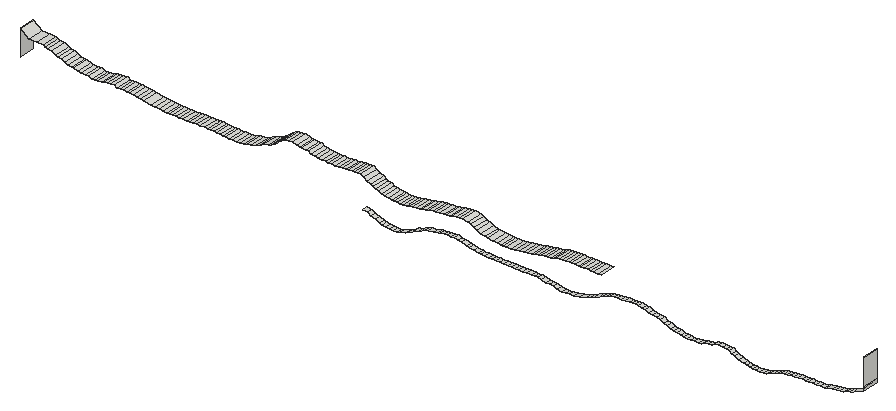
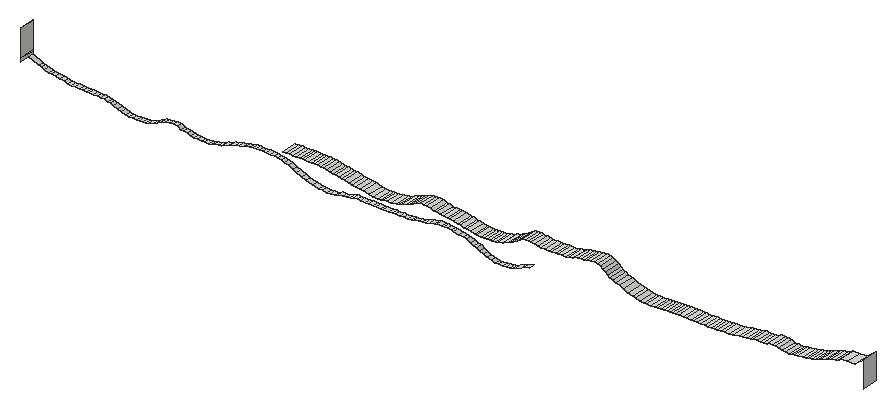
# SketchUp Ruby script. Lengths in inches.
U = 1.inch
M = Sketchup.active_model
def pt(a) = Geom::Point3d.new(a.map { |v| v * U })
def face(e, loops, mat)
  f = e.add_face(loops[0].map { |a| pt(a) })
  loops[1..].each { |l| e.add_face(l.map { |a| pt(a) }).erase! }
  f.material = f.back_material = mat if mat
  f
end
# faces: each face lists its corners as indices into pts; further lists are holes
def faces(e, pts, list, mat = nil) = list.each { |f| face(e, (f[0].is_a?(Array) ? f : [f]).map { |l| l.map { |i| pts[i] } }, mat) }
# xy, xz, yz: faces in a plane at the given z, y or x. An outline is a flat list of corners, or four numbers for a rectangle; further outlines are holes
def ring(l) = l.size == 4 ? [[l[0], l[1]], [l[2], l[1]], [l[2], l[3]], [l[0], l[3]]] : l.each_slice(2).to_a
def flat(e, list, mat, &to3) = list.each { |f| face(e, (f[0].is_a?(Array) ? f : [f]).map { |l| ring(l).map { |u, v| to3.(u, v) } }, mat) }
def xy(e, z, list, mat = nil) = flat(e, list, mat) { |x, y| [x, y, z] }
def xz(e, y, list, mat = nil) = flat(e, list, mat) { |x, z| [x, y, z] }
def yz(e, x, list, mat = nil) = flat(e, list, mat) { |y, z| [x, y, z] }
def lines(e, pts, list) = list.each { |a, b| e.add_line(pt(pts[a]), pt(pts[b])) }
# prism: a flat outline (further loops are holes) pulled along v
def prism(e, loops, v, mat = nil)
  f = face(e, loops, mat); d = Geom::Vector3d.new(v.map { |x| x * U })
  f.pushpull(f.normal.samedirection?(d) ? d.length : -d.length)
end
def box(e, o, s, mat = nil) = prism(e, [[o, [o[0] + s[0], o[1], o[2]], [o[0] + s[0], o[1] + s[1], o[2]], [o[0], o[1] + s[1], o[2]]]], [0, 0, s[2]], mat)
def at(x, y, z, deg = 0) = Geom::Transformation.translation(pt([x, y, z])) * Geom::Transformation.rotation(ORIGIN, Z_AXIS, deg.degrees)
def axes(o, x, y, z) = Geom::Transformation.new([*x, 0, *y, 0, *z, 0, *pt(o).to_a, 1])
def part(name) = M.definitions.add(name)
# library, detail: a bought-in or finely detailed component or shape, given as its bounding box
def library(name, o, s) = part(name).tap { |d| box(d.entities, o, s) }
def detail(e, o, s) = box(e.add_group.entities, o, s)
def put(e, d, t, mat = nil) = e.add_instance(d, t).tap { |i| i.material = mat if mat }
def group(e, t, mat = nil) = e.add_group.tap { |g| g.transformation = t; g.material = mat if mat }.entities
root = M.entities
xy(root,238.18,[[376.03,565.74,376.71,566.68]])
xy(root,238.62,[[342.56,565.74,343.33,566.68],[343.33,565.74,343.96,566.68],[343.96,565.74,344.72,566.68],[344.72,565.74,345.34,566.68],[345.34,565.74,346.19,566.68],
  [346.19,565.74,346.83,566.68],[346.83,565.74,347.45,566.68]])
xy(root,238.625,[[341.14,565.74,342,566.68]])
xy(root,238.89,[[396.95,565.74,397.63,566.68]])
xy(root,238.9,[[398.39,565.74,399.01,566.68],[399.01,565.74,399.78,566.68]])
xy(root,240.43,[[365.23,565.74,365.8,566.68]])
xy(root,241.68,[[283.28,565.74,283.87,568.68]])
xy(root,241.75,[[285.63,565.74,286.5,568.68],[286.5,565.74,287.12,568.68],[287.12,565.74,287.63,568.68]])
xy(root,243.05,[[358.29,565.74,358.97,568.68]])
xy(root,243.07,[[356.4375,565.74,357.02,568.68]])
xy(root,243.09,[[353.125,565.74,353.65,568.68],[353.65,565.74,354.17,568.68],[354.17,565.74,354.83,568.68],[354.83,565.74,355.28,568.68]])
yz(root,252.84,[[565.74,241.52,568.68,246.2]])
yz(root,406.85,[[565.74,240.89,565.74,241.29,568.68,241.52,568.68,240.89],[565.74,241.29,568.68,241.52,565.74,241.52],[565.74,241.52,565.74,246.27,566.4375,246.36,568.68,246.43,568.68,241.52],[565.74,246.27,565.74,246.43,568.68,246.43,566.4375,246.36]])
p = [[319.64,565.74,237.11],[319.64,566.68,237.11],[320.4,566.68,237.04],[320.4,565.74,237.04],[321.09,566.68,237.01],[321.09,565.74,237.01],
  [321.7,566.68,236.98],[321.7,565.74,236.98],[322.38,566.68,237.22],[322.38,565.74,237.22],[318.95,565.74,237.2],[318.95,566.68,237.2],
  [318.42,565.74,237.33],[318.42,566.68,237.33],[323.23,566.68,237.43],[323.23,565.74,237.43],[317.75,565.74,237.68],[317.75,566.68,237.68],
  [323.85,566.68,237.74],[323.85,565.74,237.74],[386.68,565.74,237.45],[386.68,566.68,237.45],[387.25,566.68,237.42],[387.25,565.74,237.42],
  [387.98,566.68,237.4],[387.98,565.74,237.4],[388.66,566.68,237.47],[388.66,565.74,237.47],[385.49,565.74,237.59],[385.49,566.68,237.59],
  [386.09,566.68,237.51],[386.09,565.74,237.51],[389.26,566.68,237.5625],[389.26,565.74,237.5625],[384.95,565.74,237.71],[384.95,566.68,237.71],
  [389.95,566.68,237.84],[389.95,565.74,237.84],[316.8125,565.74,237.96],[316.8125,566.68,237.96],[324.55,566.68,238.02],[324.55,565.74,238.02],
  [351.69,565.74,237.79],[351.69,566.68,237.79],[352.4,566.68,237.74],[352.4,565.74,237.74],[353.27,566.68,237.87],[353.27,565.74,237.87],
  [384.12,565.74,238],[384.12,566.68,238],[350.92,565.74,237.86],[350.92,566.68,237.86],[390.63,566.68,238.08],[390.63,565.74,238.08],
  [350.29,565.74,238.15],[350.29,566.68,238.15],[353.92,566.68,237.88],[353.92,565.74,237.88],[355.04,566.68,238.14],[355.04,565.74,238.14],
  [316.25,565.74,238.28],[316.25,566.68,238.28],[324.99,566.68,238.375],[324.99,565.74,238.375],[383.41,565.74,238.33],[383.41,566.68,238.33],
  [349.52,565.74,238.19],[349.52,566.68,238.19],[356.26,566.68,238.46],[356.26,565.74,238.46],[374.01,565.74,238.19],[374.01,566.68,238.19],
  [374.83,566.68,238.15],[374.83,565.74,238.15],[375.36,566.68,238.11],[375.36,565.74,238.11],[376.03,566.68,238.18],[376.03,565.74,238.18],
  [391.32,566.68,238.33],[391.32,565.74,238.33],[348.9,565.74,238.25],[348.9,566.68,238.25],[373.4375,565.74,238.26],[373.4375,566.68,238.26],
  [376.71,565.74,238.18],[376.71,566.68,238.18],[377.39,566.68,238.27],[377.39,565.74,238.27],[315.47,565.74,238.43],[315.47,566.68,238.43],
  [348.14,565.74,238.45],[348.14,566.68,238.45],[372.87,565.74,238.48],[372.87,566.68,238.48],[377.91,566.68,238.55],[377.91,565.74,238.55],
  [382.86,565.74,238.57],[382.86,566.68,238.57],[391.85,566.68,238.51],[391.85,565.74,238.51],[325.55,566.68,238.51],[325.55,565.74,238.51],
  [326.1875,566.68,238.76],[326.1875,565.74,238.76],[347.45,565.74,238.62],[347.45,566.68,238.62],[357.01,566.68,238.72],[357.01,565.74,238.72],
  [372.21,565.74,238.56],[372.21,566.68,238.56],[378.57,566.68,238.61],[378.57,565.74,238.61],[392.42,566.68,238.6],[392.42,565.74,238.6],
  [338.38,565.74,238.66],[338.38,566.68,238.66],[339.05,566.68,238.65],[339.05,565.74,238.65],[339.83,566.68,238.64],[339.83,565.74,238.64],
  [340.45,566.68,238.63],[340.45,565.74,238.63],[341.14,566.68,238.625],[341.14,565.74,238.625],[342,565.74,238.625],[342,566.68,238.625],
  [342.56,566.68,238.62],[342.56,565.74,238.62],[371.64,565.74,238.67],[371.64,566.68,238.67],[379.16,566.68,238.66],[379.16,565.74,238.66],
  [382.36,565.74,238.86],[382.36,566.68,238.86],[393.08,566.68,238.74],[393.08,565.74,238.74],[336.54,565.74,238.78],[336.54,566.68,238.78],
  [337.02,566.68,238.73],[337.02,565.74,238.73],[337.69,566.68,238.6875],[337.69,565.74,238.6875],[357.89,566.68,239.08],[357.89,565.74,239.08],
  [371.12,565.74,239.01],[371.12,566.68,239.01],[379.73,566.68,239.04],[379.73,565.74,239.04],[393.66,566.68,238.8],[393.66,565.74,238.8],
  [326.83,566.68,239.12],[326.83,565.74,239.12],[335.66,565.74,238.93],[335.66,566.68,238.93],[394.23,566.68,238.83],[394.23,565.74,238.83],
  [394.97,566.68,238.86],[394.97,565.74,238.86],[334.89,565.74,239.07],[334.89,566.68,239.07],[381.84,565.74,238.96],[381.84,566.68,238.96],
  [395.73,566.68,238.875],[395.73,565.74,238.875],[396.27,566.68,238.88],[396.27,565.74,238.88],[396.95,566.68,238.89],[396.95,565.74,238.89],
  [397.63,565.74,238.89],[397.63,566.68,238.89],[398.39,566.68,238.9],[398.39,565.74,238.9],[399.78,565.74,238.9],[399.78,566.68,238.9],
  [400.41,566.68,239.15],[400.41,565.74,239.15],[370.4375,565.74,239.18],[370.4375,566.68,239.18],[380.47,566.68,239.125],[380.47,565.74,239.125],
  [381.15,566.68,239.02],[381.15,565.74,239.02],[327.41,566.68,239.22],[327.41,565.74,239.22],[334.34,565.74,239.16],[334.34,566.68,239.16],
  [358.68,566.68,239.375],[358.68,565.74,239.375],[328.41,566.68,239.31],[328.41,565.74,239.31],[333.49,565.74,239.44],[333.49,566.68,239.44],
  [369.8125,565.74,239.5],[369.8125,566.68,239.5],[401.18,566.68,239.28],[401.18,565.74,239.28],[329.22,566.68,239.54],[329.22,565.74,239.54],
  [401.98,566.68,239.42],[401.98,565.74,239.42],[332.82,565.74,239.56],[332.82,566.68,239.56],[359.42,566.68,239.75],[359.42,565.74,239.75],
  [402.7,566.68,239.49],[402.7,565.74,239.49],[329.71,566.68,239.6],[329.71,565.74,239.6],[369.05,565.74,239.65],[369.05,566.68,239.65],
  [403.25,566.68,239.53],[403.25,565.74,239.53],[403.9375,566.68,239.81],[403.9375,565.74,239.81],[330.33,566.68,239.65],[330.33,565.74,239.65],
  [330.92,566.68,239.69],[330.92,565.74,239.69],[332.21,565.74,239.72],[332.21,566.68,239.72],[331.48,566.68,239.7],[331.48,565.74,239.7],
  [360.07,566.68,239.97],[360.07,565.74,239.97],[368.4375,565.74,239.8],[368.4375,566.68,239.8],[367.68,565.74,239.96],[367.68,566.68,239.96],
  [404.46,566.68,239.96],[404.46,565.74,239.96],[360.69,566.68,240.17],[360.69,565.74,240.17],[367.03,565.74,240.23],[367.03,566.68,240.23],
  [405.02,566.68,240.1],[405.02,565.74,240.1],[406.85,566.68,240.89],[406.85,565.74,240.89],[361.37,566.68,240.27],[361.37,565.74,240.27],
  [366.45,565.74,240.27],[366.45,566.68,240.27],[362.05,566.68,240.33],[362.05,565.74,240.33],[362.74,566.68,240.37],[362.74,565.74,240.37],
  [365.8,565.74,240.43],[365.8,566.68,240.43],[363.43,566.68,240.4],[363.43,565.74,240.4],[364.125,566.68,240.41],[364.125,565.74,240.41],
  [364.65,566.68,240.42],[364.65,565.74,240.42],[365.23,566.68,240.43],[365.23,565.74,240.43],[289.26,568.68,241.57],[289.8,568.68,241.53],
  [289.8,565.74,241.53],[289.26,565.74,241.57],[290.42,568.68,241.51],[290.42,565.74,241.51],[290.97,568.68,241.49],[290.97,565.74,241.49],
  [291.67,568.68,241.48],[291.67,565.74,241.48],[292.33,568.68,241.47],[292.33,565.74,241.47],[292.9,568.68,241.46],[292.9,565.74,241.46],
  [293.61,568.68,241.6],[293.61,565.74,241.6],[339.98,568.68,241.56],[340.58,568.68,241.51],[340.58,565.74,241.51],[339.98,565.74,241.56],
  [341.03,568.68,241.48],[341.03,565.74,241.48],[341.55,568.68,241.46],[341.55,565.74,241.46],[342.42,568.68,241.51],[342.42,565.74,241.51],
  [343.14,568.68,241.59],[343.14,565.74,241.59],[288.65,568.68,241.66],[288.65,565.74,241.66],[294.34,568.68,241.85],[294.34,565.74,241.85],
  [338.16,568.68,241.78],[339.21,568.68,241.63],[339.21,565.74,241.63],[338.16,565.74,241.78],[344.08,568.68,241.82],[344.08,565.74,241.82],
  [279.62,568.68,241.75],[280.07,568.68,241.74],[280.07,565.74,241.74],[279.62,565.74,241.75],[280.62,568.68,241.72],[280.62,565.74,241.72],
  [281.25,568.68,241.71],[281.25,565.74,241.71],[281.88,568.68,241.7],[281.88,565.74,241.7],[282.61,568.68,241.69],[282.61,565.74,241.69],
  [283.28,568.68,241.68],[283.28,565.74,241.68],[283.87,568.68,241.68],[284.36,568.68,241.67],[284.36,565.74,241.67],[283.87,565.74,241.68],
  [285.0625,568.68,241.74],[285.0625,565.74,241.74],[285.63,568.68,241.75],[285.63,565.74,241.75],[287.63,568.68,241.75],[288.12,568.68,241.67],
  [288.12,565.74,241.67],[287.63,565.74,241.75],[277.43,568.68,241.89],[278.25,568.68,241.83],[278.25,565.74,241.83],[277.43,565.74,241.89],
  [278.85,568.68,241.78],[278.85,565.74,241.78],[295.01,568.68,241.91],[295.01,565.74,241.91],[320.64,568.68,241.89],[321.1,568.68,241.85],
  [321.1,565.74,241.85],[320.64,565.74,241.89],[321.62,568.68,241.8125],[321.62,565.74,241.8125],[322.13,568.68,241.79],[322.13,565.74,241.79],
  [322.71,568.68,241.78],[322.71,565.74,241.78],[323.38,568.68,241.91],[323.38,565.74,241.91],[337.67,568.68,241.89],[337.67,565.74,241.89],
  [344.86,568.68,241.87],[344.86,565.74,241.87],[276.66,568.68,241.96],[276.66,565.74,241.96],[295.91,568.68,242.1],[295.91,565.74,242.1],
  [320.08,568.68,241.96],[320.08,565.74,241.96],[323.85,568.68,241.93],[323.85,565.74,241.93],[324.52,568.68,242.09],[324.52,565.74,242.09],
  [337.03,568.68,242.14],[337.03,565.74,242.14],[345.625,568.68,241.98],[345.625,565.74,241.98],[275.49,568.68,242.24],[275.49,565.74,242.24],
  [319.4,568.68,242.11],[319.4,565.74,242.11],[346.24,568.68,242.02],[346.24,565.74,242.02],[346.89,568.68,242.19],[346.89,565.74,242.19],
  [296.68,568.68,242.46],[296.68,565.74,242.46],[318.8,568.68,242.21],[318.8,565.74,242.21],[325.29,568.68,242.2],[325.29,565.74,242.2],
  [336.27,568.68,242.39],[336.27,565.74,242.39],[274.82,568.68,242.34],[274.82,565.74,242.34],[318.29,568.68,242.51],[318.29,565.74,242.51],
  [325.79,568.68,242.24],[325.79,565.74,242.24],[326.4,568.68,242.42],[326.4,565.74,242.42],[347.59,568.68,242.38],[347.59,565.74,242.38],
  [274.16,568.68,242.38],[274.16,565.74,242.38],[273.5,568.68,242.48],[273.5,565.74,242.48],[326.95,568.68,242.47],[326.95,565.74,242.47],
  [335.65,568.68,242.65],[335.65,565.74,242.65],[348.08,568.68,242.4375],[348.08,565.74,242.4375],[348.6,568.68,242.48],[348.6,565.74,242.48],
  [265.32,568.68,242.68],[265.99,568.68,242.51],[265.99,565.74,242.51],[265.32,565.74,242.68],[266.51,568.68,242.46],[266.51,565.74,242.46],
  [267.05,568.68,242.58],[267.05,565.74,242.58],[272.86,568.68,242.57],[272.86,565.74,242.57],[297.38,568.68,242.78],[297.38,565.74,242.78],
  [317.7,568.68,242.68],[317.7,565.74,242.68],[327.7,568.68,242.71],[327.7,565.74,242.71],[349.26,568.68,242.58],[349.26,565.74,242.58],
  [267.68,568.68,242.57],[267.68,565.74,242.57],[268.31,568.68,242.81],[268.31,565.74,242.81],[270.08,568.68,242.92],[270.51,568.68,242.625],
  [270.51,565.74,242.625],[270.08,565.74,242.92],[271.12,568.68,242.65],[271.12,565.74,242.65],[271.67,568.68,242.62],[271.67,565.74,242.62],
  [272.3,568.68,242.58],[272.3,565.74,242.58],[335.1,568.68,242.9375],[335.1,565.74,242.9375],[349.79,568.68,242.61],[349.79,565.74,242.61],
  [350.375,568.68,242.77],[350.375,565.74,242.77],[263.97,568.68,242.78],[264.78,568.68,242.73],[264.78,565.74,242.73],[263.97,565.74,242.78],
  [317.2,568.68,242.875],[317.2,565.74,242.875],[328.34,568.68,242.78],[328.34,565.74,242.78],[262.67,568.68,243.06],[263.39,568.68,242.85],
  [263.39,565.74,242.85],[262.67,565.74,243.06],[268.88,568.68,242.86],[268.88,565.74,242.86],[298.15,568.68,242.97],[298.15,565.74,242.97],
  [328.82,568.68,242.82],[328.82,565.74,242.82],[329.51,568.68,242.85],[329.51,565.74,242.85],[350.83,568.68,242.95],[350.83,565.74,242.95],
  [269.44,568.68,242.89],[269.44,565.74,242.89],[316.81,568.68,243.09],[316.81,565.74,243.09],[330.21,568.68,242.87],[330.21,565.74,242.87],
  [330.76,568.68,243.02],[330.76,565.74,243.02],[334.53,568.68,243.14],[334.53,565.74,243.14],[298.68,568.68,243.23],[298.68,565.74,243.23],
  [331.38,568.68,243.05],[331.38,565.74,243.05],[351.39,568.68,243.01],[351.39,565.74,243.01],[351.9,568.68,243.05],[351.9,565.74,243.05],
  [352.47,568.68,243.08],[352.47,565.74,243.08],[261.6,568.68,243.3],[262.1875,568.68,243.14],[262.1875,565.74,243.14],[261.6,565.74,243.3],
  [316.2,568.68,243.43],[316.2,565.74,243.43],[331.93,568.68,243.29],[331.93,565.74,243.29],[333.76,568.68,243.42],[333.76,565.74,243.42],
  [353.125,568.68,243.09],[353.125,565.74,243.09],[355.28,568.68,243.09],[355.85,568.68,243.08],[355.85,565.74,243.08],[355.28,565.74,243.09],
  [356.4375,568.68,243.07],[356.4375,565.74,243.07],[357.02,568.68,243.07],[357.68,568.68,243.0625],[357.68,565.74,243.0625],[357.02,565.74,243.07],
  [358.29,568.68,243.05],[358.29,565.74,243.05],[299.08,568.68,243.48],[299.08,565.74,243.48],[260.96,568.68,243.48],[260.96,565.74,243.48],
  [332.61,568.68,243.35],[332.61,565.74,243.35],[315.66,568.68,243.8],[315.66,565.74,243.8],[333.16,568.68,243.39],[333.16,565.74,243.39],
  [260.44,568.68,243.79],[260.44,565.74,243.79],[299.6,568.68,243.72],[299.6,565.74,243.72],[299.9375,568.68,244.12],[299.9375,565.74,244.12],
  [259.78,568.68,243.95],[259.78,565.74,243.95],[315.06,568.68,244.18],[315.06,565.74,244.18],[259.26,568.68,244.11],[259.26,565.74,244.11],
  [307.88,568.68,243.99],[308.6,568.68,243.95],[308.6,565.74,243.95],[307.88,565.74,243.99],[309.1,568.68,243.93],[309.1,565.74,243.93],
  [309.79,568.68,243.91],[309.79,565.74,243.91],[310.36,568.68,243.89],[310.36,565.74,243.89],[311.06,568.68,243.88],[311.06,565.74,243.88],
  [311.71,568.68,243.94],[311.71,565.74,243.94],[312.35,568.68,243.95],[312.35,565.74,243.95],[312.91,568.68,244.1],[312.91,565.74,244.1],
  [306.7,568.68,244.11],[307.26,568.68,244.04],[307.26,565.74,244.04],[306.7,565.74,244.11],[258.59,568.68,244.41],[258.59,565.74,244.41],
  [300.41,568.68,244.39],[300.41,565.74,244.39],[305.95,568.68,244.25],[305.95,565.74,244.25],[313.54,568.68,244.13],[313.54,565.74,244.13],
  [314.02,568.68,244.15],[314.02,565.74,244.15],[314.54,568.68,244.17],[314.54,565.74,244.17],[305.49,568.68,244.51],[305.49,565.74,244.51],
  [257.83,568.68,244.54],[257.83,565.74,244.54],[300.89,568.68,244.73],[300.89,565.74,244.73],[257.27,568.68,244.61],[257.27,565.74,244.61],
  [304.34,568.68,244.67],[304.95,568.68,244.55],[304.95,565.74,244.55],[304.34,565.74,244.67],[257.05,568.68,244.92],[257.05,565.74,244.92],
  [301.375,568.68,244.87],[301.375,565.74,244.87],[303.29,568.68,244.81],[303.86,568.68,244.7],[303.86,565.74,244.7],[303.29,565.74,244.81],
  [302.64,568.68,245.01],[302.64,565.74,245.01],[254.41,568.68,244.96],[255.8,568.68,244.9375],[255.8,565.74,244.9375],[254.41,565.74,244.96],
  [301.96,568.68,244.95],[301.96,565.74,244.95],[252.84,568.68,246.2],[252.84,565.74,246.2]]
faces(root,p,[[0,1,2,3],[3,2,4,5],[5,4,6,7],[7,6,8,9],[10,11,1,0],[12,13,11,10],[9,8,14,15],[16,17,13,12],
  [15,14,18,19],[20,21,22,23],[23,22,24,25],[25,24,26,27],[28,29,30,31],[31,30,21,20],[27,26,32,33],[34,35,29,28],
  [33,32,36,37],[38,39,17,16],[19,18,40,41],[42,43,44,45],[45,44,46,47],[48,49,35,34],[50,51,43,42],[37,36,52,53],
  [54,55,51,50],[47,46,56,57],[57,56,58,59],[60,61,39,38],[41,40,62,63],[64,65,49,48],[66,67,55,54],[59,58,68,69],
  [70,71,72,73],[73,72,74,75],[75,74,76,77],[53,52,78,79],[80,81,67,66],[82,83,71,70],[84,85,86,87],[88,89,61,60],
  [90,91,81,80],[92,93,83,82],[87,86,94,95],[96,97,65,64],[79,78,98,99],[63,62,100,101],[101,100,102,103],[104,105,91,90],
  [69,68,106,107],[108,109,93,92],[95,94,110,111],[99,98,112,113],[114,115,116,117],[117,116,118,119],[119,118,120,121],[121,120,122,123],
  [124,125,126,127],[128,129,109,108],[111,110,130,131],[132,133,97,96],[113,112,134,135],[136,137,138,139],[139,138,140,141],[141,140,115,114],
  [107,106,142,143],[144,145,129,128],[131,130,146,147],[135,134,148,149],[103,102,150,151],[152,153,137,136],[149,148,154,155],[155,154,156,157],
  [158,159,153,152],[160,161,133,132],[157,156,162,163],[163,162,164,165],[165,164,166,167],[168,169,170,171],[172,173,174,175],[176,177,145,144],
  [147,146,178,179],[179,178,180,181],[181,180,161,160],[151,150,182,183],[184,185,159,158],[143,142,186,187],[183,182,188,189],[190,191,185,184],
  [192,193,177,176],[175,174,194,195],[189,188,196,197],[195,194,198,199],[200,201,191,190],[187,186,202,203],[199,198,204,205],[197,196,206,207],
  [208,209,193,192],[205,204,210,211],[211,210,212,213],[207,206,214,215],[215,214,216,217],[218,219,201,200],[217,216,220,221],[221,220,219,218],
  [203,202,222,223],[224,225,209,208],[226,227,225,224],[213,212,228,229],[223,222,230,231],[232,233,227,226],[229,228,234,235],[235,234,236,237],
  [231,230,238,239],[240,241,233,232],[239,238,242,243],[243,242,244,245],[246,247,241,240],[245,244,248,249],[249,248,250,251],[251,250,252,253],
  [253,252,254,255],[256,257,258,259],[257,260,261,258],[260,262,263,261],[262,264,265,263],[264,266,267,265],[266,268,269,267],[268,270,271,269],
  [272,273,274,275],[273,276,277,274],[276,278,279,277],[278,280,281,279],[280,282,283,281],[284,256,259,285],[270,286,287,271],[288,289,290,291],
  [289,272,275,290],[282,292,293,283],[294,295,296,297],[295,298,299,296],[298,300,301,299],[300,302,303,301],[302,304,305,303],[304,306,307,305],
  [308,309,310,311],[309,312,313,310],[312,314,315,313],[316,317,318,319],[317,284,285,318],[320,321,322,323],[321,324,325,322],[324,294,297,325],
  [286,326,327,287],[328,329,330,331],[329,332,333,330],[332,334,335,333],[334,336,337,335],[336,338,339,337],[340,288,291,341],[292,342,343,293],
  [344,320,323,345],[326,346,347,327],[348,328,331,349],[338,350,351,339],[350,352,353,351],[354,340,341,355],[342,356,357,343],[358,344,345,359],
  [360,348,349,361],[356,362,363,357],[362,364,365,363],[346,366,367,347],[368,360,361,369],[352,370,371,353],[372,354,355,373],[374,358,359,375],
  [376,368,369,377],[370,378,379,371],[378,380,381,379],[364,382,383,365],[384,374,375,385],[386,384,385,387],[380,388,389,381],[390,372,373,391],
  [382,392,393,383],[392,394,395,393],[396,397,398,399],[397,400,401,398],[400,402,403,401],[404,386,387,405],[366,406,407,367],[408,376,377,409],
  [388,410,411,389],[394,412,413,395],[402,414,415,403],[414,416,417,415],[418,419,420,421],[419,422,423,420],[422,424,425,423],[424,426,427,425],
  [426,404,405,427],[428,390,391,429],[412,430,431,413],[430,432,433,431],[434,435,436,437],[435,396,399,436],[438,408,409,439],[410,440,441,411],
  [442,443,444,445],[443,434,437,444],[416,446,447,417],[406,448,449,407],[440,450,451,441],[450,452,453,451],[432,454,455,433],[446,456,457,447],
  [456,418,421,457],[458,438,439,459],[452,460,461,453],[460,462,463,461],[464,428,429,465],[448,466,467,449],[462,468,469,463],[454,470,471,455],
  [470,472,473,471],[472,474,475,473],[476,477,478,479],[477,442,445,478],[480,458,459,481],[468,482,483,469],[484,464,465,485],[474,486,487,475],
  [488,489,490,491],[489,492,493,490],[494,495,496,497],[495,498,499,496],[466,500,501,467],[502,476,479,503],[482,504,505,483],[506,480,481,507],
  [504,508,509,505],[508,484,485,509],[510,502,503,511],[500,512,513,501],[512,514,515,513],[516,510,511,517],[518,506,507,519],[520,516,517,521],
  [522,523,524,525],[523,526,527,524],[526,528,529,527],[528,530,531,529],[530,532,533,531],[532,534,535,533],[534,536,537,535],[536,538,539,537],
  [540,541,542,543],[541,522,525,542],[544,520,521,545],[514,546,547,515],[548,540,543,549],[538,550,551,539],[550,552,553,551],[552,554,555,553],
  [554,518,519,555],[556,548,549,557],[558,544,545,559],[546,560,561,547],[562,558,559,563],[564,565,566,567],[565,556,557,566],[568,562,563,569],
  [560,570,571,561],[572,573,574,575],[573,564,567,574],[576,572,575,577],[578,579,580,581],[579,568,569,580],[570,582,583,571],[582,576,577,583],
  [584,578,581,585]])
